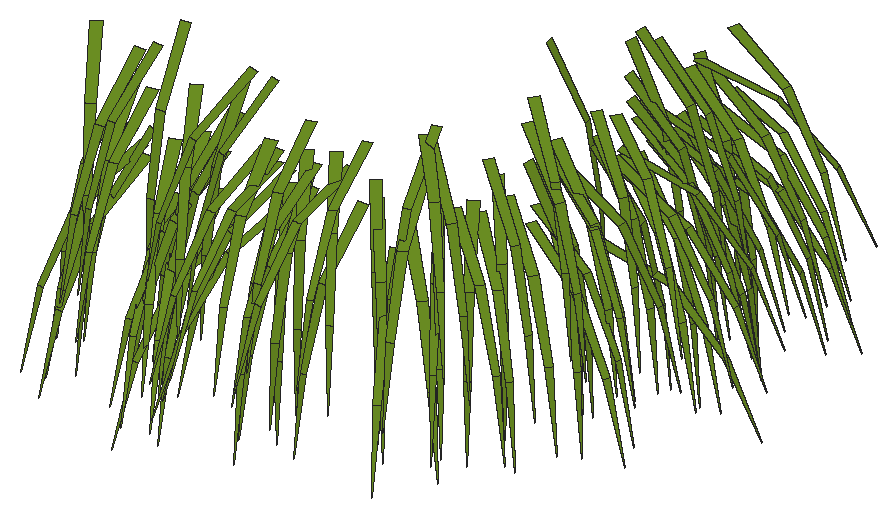
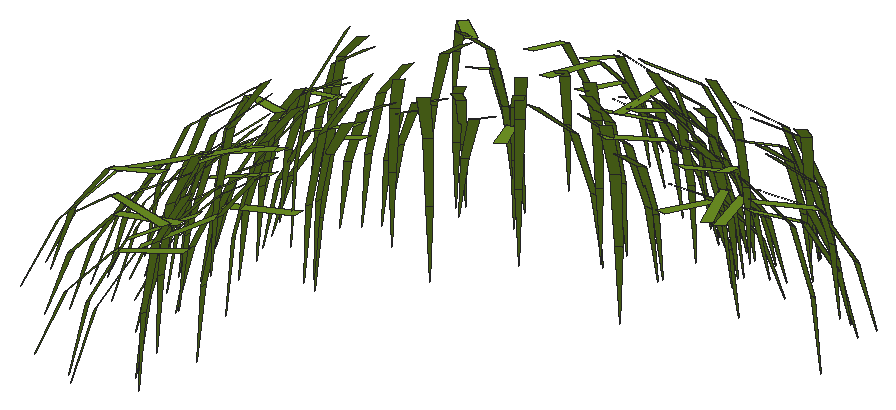
# SketchUp Ruby script. Lengths in inches.
U = 1.inch
M = Sketchup.active_model
def pt(a) = Geom::Point3d.new(a.map { |v| v * U })
def face(e, loops, mat)
  f = e.add_face(loops[0].map { |a| pt(a) })
  loops[1..].each { |l| e.add_face(l.map { |a| pt(a) }).erase! }
  f.material = f.back_material = mat if mat
  f
end
# faces: each face lists its corners as indices into pts; further lists are holes
def faces(e, pts, list, mat = nil) = list.each { |f| face(e, (f[0].is_a?(Array) ? f : [f]).map { |l| l.map { |i| pts[i] } }, mat) }
# xy, xz, yz: faces in a plane at the given z, y or x. An outline is a flat list of corners, or four numbers for a rectangle; further outlines are holes
def ring(l) = l.size == 4 ? [[l[0], l[1]], [l[2], l[1]], [l[2], l[3]], [l[0], l[3]]] : l.each_slice(2).to_a
def flat(e, list, mat, &to3) = list.each { |f| face(e, (f[0].is_a?(Array) ? f : [f]).map { |l| ring(l).map { |u, v| to3.(u, v) } }, mat) }
def xy(e, z, list, mat = nil) = flat(e, list, mat) { |x, y| [x, y, z] }
def xz(e, y, list, mat = nil) = flat(e, list, mat) { |x, z| [x, y, z] }
def yz(e, x, list, mat = nil) = flat(e, list, mat) { |y, z| [x, y, z] }
def lines(e, pts, list) = list.each { |a, b| e.add_line(pt(pts[a]), pt(pts[b])) }
# prism: a flat outline (further loops are holes) pulled along v
def prism(e, loops, v, mat = nil)
  f = face(e, loops, mat); d = Geom::Vector3d.new(v.map { |x| x * U })
  f.pushpull(f.normal.samedirection?(d) ? d.length : -d.length)
end
def box(e, o, s, mat = nil) = prism(e, [[o, [o[0] + s[0], o[1], o[2]], [o[0] + s[0], o[1] + s[1], o[2]], [o[0], o[1] + s[1], o[2]]]], [0, 0, s[2]], mat)
def at(x, y, z, deg = 0) = Geom::Transformation.translation(pt([x, y, z])) * Geom::Transformation.rotation(ORIGIN, Z_AXIS, deg.degrees)
def axes(o, x, y, z) = Geom::Transformation.new([*x, 0, *y, 0, *z, 0, *pt(o).to_a, 1])
def part(name) = M.definitions.add(name)
# library, detail: a bought-in or finely detailed component or shape, given as its bounding box
def library(name, o, s) = part(name).tap { |d| box(d.entities, o, s) }
def detail(e, o, s) = box(e.add_group.entities, o, s)
def put(e, d, t, mat = nil) = e.add_instance(d, t).tap { |i| i.material = mat if mat }
def group(e, t, mat = nil) = e.add_group.tap { |g| g.transformation = t; g.material = mat if mat }.entities
root = M.entities
M.materials.add("[0061_OliveDrab]").color = [107, 142, 35]
p = [[570.33,4.46,549.35],[570.13,4.36,549.35],[570.3,4.27,546.73],[578.04,13.58,549.32],[578.01,13.38,549.32],[578.3,13.43,546.71],
  [567.76,2.63,549.36],[567.58,2.6,549.36],[567.8,2,546.81],[577.62,8.9,549.64],[577.5,8.72,549.64],[577.875,8.6,547.04],
  [578.36,15.74,549.62],[578.36,15.53,549.62],[578.73,15.64,547.02],[567.34,1.68,549.49],[567.14,1.69,549.49],[567.19,0.69,547.06],
  [570.32,2.78,549.65],[570.15,2.71,549.65],[570.51,2.05,547.13],[563.88,3.65,549.66],[563.7,3.71,549.66],[563.71,3.4,547.05],
  [575.6,6.45,549.68],[575.43,6.34,549.68],[575.66,6.18,547.07],[580.17,12.39,549.47],[580.18,12.16,549.47],[581.41,12.33,547.16],
  [578.24,15.81,549.85],[578.24,15.61,549.85],[578.58,15.7,547.25],[579.03,17.18,549.77],[579.1,16.98,549.77],[579.73,17.33,547.24],
  [564.12,2.25,549.77],[563.9,2.27,549.77],[563.95,1.45,547.28],[577.73,16.7,549.91],[577.68,16.5,549.91],[577.91,16.55,547.29],
  [572.05,3.42,550],[571.84,3.41,550],[571.97,2.97,547.42],[579.04,12.85,549.91],[578.99,12.68,549.91],[579.77,12.5625,547.41],
  [570.27,3.16,550.09],[570.04,3.16,550.09],[570.14,2.75,547.49],[579.09,17.45,550.14],[579.13,17.26,550.14],[579.69,17.49,547.59],
  [574.92,3.2,550.09],[574.74,3.09,550.09],[575.37,2.26,547.68],[573.54,4.96,550.3],[573.39,4.83,550.3],[573.6,4.74,547.68],
  [579.03,14.57,550.21],[579.03,14.34,550.21],[579.68,14.45,547.66],[579.96,17.4,550.125],[579.97,17.18,550.125],[581.05,17.32,547.74],
  [563.45,2.23,550.33],[563.23,2.28,550.33],[563.19,1.55,547.81],[564.05,2.47,550.34],[563.83,2.46,550.34],[563.98,1.71,547.82],
  [575.86,4.53,550.27],[575.72,4.36,550.27],[576.51,3.82,547.83],[579.09,8.36,550.21],[579.02,8.16,550.21],[580,7.93,547.79],
  [577.9,12.36,550.37],[577.94,12.15,550.37],[578.17,12.29,547.76],[567.2,1.79,550.24],[567.03,1.72,550.24],[567.6,0.59,547.95],
  [577.34,6.16,550.41],[577.21,5.99,550.41],[577.84,5.64,547.88],[578.93,9.05,550.4375],[578.89,8.87,550.4375],[579.62,8.8,547.92],
  [577.34,9.68,550.47],[577.31,9.46,550.47],[577.53,9.54,547.85],[566.8,2.1,550.51],[566.58,2.11,550.51],[566.67,1.24,548.03],
  [574.41,4.08,550.53],[574.26,3.95,550.53],[574.7,3.59,547.97],[576.52,6.95,550.65],[576.37,6.82,550.65],[576.66,6.65,548.04],
  [577.18,9.46,550.57],[577.16,9.24,550.57],[577.36,9.33,547.96],[579.02,11.88,550.44],[578.93,11.69,550.44],[579.76,11.43,547.96],
  [568.04,1.92,550.33],[567.86,1.82,550.33],[568.57,0.69,548.07],[571.08,3.375,550.67],[570.87,3.3125,550.67],[571.1,2.95,548.08],
  [577.92,7.24,550.63],[577.8,7.05,550.63],[578.45,6.78,548.1],[571.24,4.2,550.8125],[571.05,4.09,550.8125],[571.27,3.94,548.2],
  [567.06,2.41,550.78],[566.84,2.42,550.78],[566.92,1.71,548.25],[567.51,2.95,550.78],[567.3,2.88,550.78],[567.63,2.25,548.25],
  [575.84,4.57,550.78],[575.68,4.46,550.78],[576.23,3.84,548.28],[577.21,5.73,550.75],[577.09,5.55,550.75],[577.85,5.18,548.26],
  [578.26,11.375,550.86],[578.19,11.16,550.86],[578.6,11.15,548.27],[579.89,13.19,550.68],[579.88,12.99,550.68],[581.01,13.0625,548.31],
  [575.91,4.82,550.91],[575.76,4.7,550.91],[576.28,4.23,548.38],[577.45,16.27,551.05],[577.38,16.07,551.05],[577.59,16.12,548.43],
  [568.88,1.85,550.85],[568.68,1.89,550.85],[568.5625,0.79,548.47],[567.23,2.48,550.98],[567.05,2.375,550.98],[567.6,1.55,548.55],
  [578.25,14.02,551.08],[578.25,13.8,551.08],[578.57,13.9,548.48],[563.69,3.07,551.16],[563.5,3.06,551.16],[563.61,2.66,548.5625],
  [567.2,3.62,551.26],[566.99,3.67,551.26],[567.03,3.31,548.66],[577.01,7.42,551.26],[576.92,7.25,551.26],[577.35,7.14,548.67],
  [568.85,2.55,551.31],[568.64,2.57,551.31],[568.68,1.82,548.79],[578.97,10.91,551.37],[578.99,10.6875,551.37],[579.7,10.84,548.84],
  [579.76,12.26,551.29],[579.73,12.05,551.29],[580.64,12.02,548.82],[568.88,2.13,551.35],[568.6875,2.17,551.35],[568.61,1.24,548.89],
  [567.03,3.29,551.45],[566.85,3.32,551.45],[566.89,2.92,548.85],[577.92,11.11,551.53],[577.83,10.93,551.53],[578.16,10.88,548.93],
  [579.27,13.67,551.38],[579.25,13.47,551.38],[580.13,13.52,548.91],[578.53,14,551.52],[578.55,13.8,551.52],[578.97,13.9375,548.9375],
  [579.17,15.17,551.45],[579.22,14.96,551.45],[579.92,15.26,548.9375],[580,17.125,551.27],[579.98,16.91,551.27],[581.02,16.92,548.86],
  [564.84,2.89,551.65],[564.66,2.84,551.65],[564.93,2.27,549.11],[569.875,2.55,551.78],[569.66,2.49,551.78],[569.96,1.86,549.25],
  [574.83,3.89,551.78],[574.62,3.81,551.78],[575,3.21,549.25],[578.37,9.35,551.75],[578.28,9.15,551.75],[578.79,9.04,549.18],
  [579.8125,13.99,551.58],[579.85,13.8,551.58],[580.83,14.1,549.16],[579.35,16.93,551.68],[579.34,16.72,551.68],[580.25,16.76,549.22],
  [570.17,4.88,551.93],[569.89,4.74,551.93],[578.9,9.24,551.86],[578.83,9.05,551.86],[579.56,8.9,549.34],[577.36,13.74,551.85],
  [577.3125,13.47,551.85],[567.56,3.85,551.68],[567.3,3.79,551.68],[573,3.43,551.9],[572.84,3.31,551.9],[573.31,2.83,549.36],
  [567.93,4.15,552.05],[567.72,4.12,552.05],[567.85,3.91,549.43],[579.5625,15.49,551.92],[579.6,15.3,551.92],[580.44,15.57,549.45],
  [565.15,2.36,551.98],[564.95,2.32,551.98],[565.18,1.57,549.47],[567.47,3.41,551.45],[567.19,3.43,551.45],[579.15,8.9,551.9375],
  [579.07,8.72,551.9375],[579.94,8.43,549.48],[578.25,12.35,551.27],[578.27,12.03,551.27],[568.58,1.87,551.98],[568.38,1.87,551.98],
  [568.47,0.83,549.57],[571.04,2.12,552.05],[570.85,2.09,552.05],[571.08,1.27,549.57],[569.88,4.01,551.92],[569.63,3.92,551.92],
  [576.94,9.39,552.125],[576.78,9.13,552.125],[578.24,13.96,552.15],[578.25,13.73,552.15],[578.61,13.86,549.55],[579.3,15.5,552.09],
  [579.25,15.28,552.09],[580.11,15.19,549.61],[577.51,15.78,552.1],[577.51,15.47,552.1],[567.72,3.3,552.25],[567.53,3.1875,552.25],
  [567.92,2.75,549.69],[564.12,4.32,552.1875],[563.87,4.39,552.1875],[575.28,6.99,552.23],[575.04,6.83,552.23],[564.27,3.68,551.97],
  [563.96,3.7,551.97],[576.11,5.64,552.37],[575.99,5.46,552.37],[576.54,5.2,549.8125],[577.76,16.75,552.03],[577.87,16.48,552.03],
  [577.76,13.24,552.18],[577.7,12.99,552.18],[577.3,13.92,552.56],[577.26,13.7,552.56],[577.51,13.77,549.95],[577.45,15.88,552.35],
  [577.44,15.59,552.35],[577.18,16.88,552.47],[577.11,16.61,552.47],[572.03,4.39,552.44],[571.74,4.375,552.44],[574.23,4.7,552.625],
  [574.04,4.65,552.625],[574.25,4.22,550.04],[578.01,8.41,552.54],[577.92,8.22,552.54],[578.48,8.06,549.98],[574.06,4.7,552.0625],
  [573.8,4.55,552.0625],[570.34,4.08,552.54],[570.02,4.09,552.54],[580.23,16.78,552.32],[580.16,16.58,552.32],[581.52,16.26,550.09],
  [577.88,17.22,552.46],[577.94,16.95,552.46],[578.2,17.39,552.07],[578.21,17.09,552.07],[566.47,3.625,551.98],[566.23,3.52,551.98],
  [564.25,2.79,552.69],[564.04,2.77,552.69],[564.21,2.07,550.17],[564.45,3.16,552.78],[564.26,3.17,552.78],[564.35,2.69,550.2],
  [567.99,3.61,552.84],[567.82,3.65,552.84],[567.82,3.25,550.25],[577.5625,8.9375,552.27],[577.47,8.66,552.27],[577.82,14.62,552.53],
  [577.8125,14.3,552.53],[571.61,1.91,552.72],[571.4,1.9,552.72],[571.53,0.78,550.35],[567.13,3.73,552],[566.88,3.6,552],
  [563.79,3.59,552.55],[563.48,3.65,552.55],[564.02,3.81,552.6],[563.71,3.79,552.6],[565.64,4.52,552.95],[565.45,4.47,552.95],
  [565.6,4.25,550.34],[574.73,5.58,552.4],[574.52,5.34,552.4],[573.21,5.41,552.86],[573,5.22,552.86],[577.43,8.59,552.91],
  [577.32,8.42,552.91],[577.77,8.25,550.33],[571.09,2.58,552.96],[570.89,2.52,552.96],[571.1875,1.82,550.45],[564.13,3.57,552.9375],
  [563.95,3.45,552.9375],[564.34,3.07,550.37],[576.31,7.02,552.67],[576.12,6.78,552.67],[577.6,9.39,552.67],[577.54,9.13,552.67],
  [579.36,10.85,552.79],[579.26,10.68,552.79],[580.19,10.24,550.375],[577.74,12.5,552.65],[577.62,12.24,552.65],[577.25,12.31,552.91],
  [577.3,12,552.91],[578.61,14.86,552.96],[578.59,14.67,552.96],[579.18,14.7,550.4],[569.75,1.36,552.77],[569.5625,1.34,552.77],
  [569.84,0,550.53],[572.87,2.68,553.01],[572.6875,2.63,553.01],[572.99,1.8125,550.53],[566.88,3.61,552.66],[566.58,3.61,552.66],
  [573.7,4.96,552.9],[573.49,4.78,552.9],[576.79,9.8125,553.03],[576.74,9.5,553.03],[576.02,7.55,553.16],[575.8125,7.36,553.16],
  [576.83,7.97,552.91],[576.66,7.69,552.91],[576.66,9.55,553.14],[576.63,9.24,553.14],[575.96,11.96,553.17],[576,11.77,553.17],
  [576.13,11.89,550.55],[578.12,14.51,553.21],[578.1,14.29,553.21],[578.58,14.35,550.63],[579.6,17.55,553.04],[579.55,17.33,553.04],
  [580.54,17.22,550.61],[579.57,18.16,552.93],[579.64,17.98,552.93],[580.67,18.46,550.57],[567.04,3.12,553.25],[566.86,3.16,553.25],
  [566.8,2.54,550.7],[566.84,2.64,551.16],[570.84,4.26,553.13],[570.56,4.17,553.13],[576.01,6.57,552.93],[575.85,6.32,552.93],
  [578.14,13.27,552.64],[578.13,12.99,552.64],[567.16,3.73,553.05],[566.85,3.74,553.05],[567.15,4.125,553.11],[566.85,4.02,553.11],
  [570.95,4.75,553.36],[570.6875,4.59,553.36],[575.06,5.74,552.99],[574.84,5.58,552.99],[569.26,3.55,552.82],[568.98,3.61,552.82],
  [575.11,5.83,553.2],[574.9,5.65,553.2],[577.45,11.69,553.34],[577.35,11.38,553.34],[566.52,3.93,553.05],[566.25,3.79,553.05],
  [576.98,16.48,553.625],[576.89,16.2,553.625],[577.47,14.09,553.59],[577.46,13.78,553.59],[563.6875,4,553.61],[563.43,3.99,553.61],
  [576.18,4.51,553.62],[576.02,4.36,553.62],[576.8125,3.71,551.2],[569.21,3.65,553.47],[568.93,3.7,553.47],[569.01,3.85,553.59],
  [568.71,3.88,553.59],[567.41,4.375,553.77],[567.11,4.4375,553.77],[576.21,7.87,553.72],[576.09,7.625,553.72],[575.7,12.27,551.85],
  [575.71,11.88,551.85],[578.18,12.55,553.36],[578.13,12.25,553.36],[578.25,17.33,553.22],[578.22,17.03,553.22],[567.19,4.16,553.92],
  [566.93,4.2,553.92],[577.65,10.875,553.64],[577.67,10.5625,553.64],[577.85,13.79,553.59],[577.84,13.51,553.59],[567.64,5.95,552.1],
  [567.3,5.97,552.1],[577.24,11.48,554.04],[577.12,11.23,554.04],[577.57,13.96,553.97],[577.59,13.67,553.97],[577.84,14.85,553.69],
  [577.91,14.57,553.69],[578.12,13.6875,553.57],[578.18,13.42,553.57],[564.53,4.04,553.99],[564.27,3.97,553.99],[567.16,5.99,553.14],
  [566.84,5.93,553.14],[577.89,17.09,553.86],[577.87,16.79,553.86],[569.55,3.83,554.05],[569.25,3.74,554.05],[574.34,5.15,554.03],
  [574.06,5.02,554.03],[577.39,9.84,554.14],[577.26,9.5625,554.14],[572.3,4.51,554.19],[572.06,4.34,554.19],[569.125,6.02,553.4375],
  [568.82,5.9,553.4375],[569.64,6.04,554.22],[569.3,5.875,554.22],[569.75,5.8125,553.77],[577.72,9.59,554.02],[577.6,9.35,554.02],
  [577.61,9.72,554.1],[577.52,9.45,554.1],[575.74,14.08,553.88],[575.68,13.74,553.88],[578.03,15.22,554.04],[578.09,14.95,554.04],
  [568.64,3.55,554],[568.36,3.55,554],[564.96,3.76,554.19],[564.67,3.71,554.19],[565.49,6.02,552.42],[565.2,5.9,552.42],
  [565.94,6.04,552.37],[565.64,5.88,552.37],[564.47,5.95,553.28],[564.09,5.97,553.28],[567.89,4.74,554.6],[567.59,4.7,554.6],
  [575.64,16,553.38],[575.77,15.66,553.38],[570.84,3.65,554.18],[570.57,3.61,554.18],[572.79,6.85,552.86],[572.47,6.66,552.86],
  [575.49,10.37,554.08],[575.29,10.05,554.08],[577.37,13.97,554.63],[577.38,13.65,554.63],[577.89,15.89,554.27],[577.8125,15.58,554.27],
  [575.7,15.8,554],[575.71,15.43,554],[575.7,17.35,552.87],[575.71,16.98,552.87],[564.61,5.91,554.21],[564.31,6,554.21],
  [574.46,8.25,554.38],[574.17,8.05,554.38],[575.75,13.8125,553.76],[575.66,13.51,553.76],[567.16,4.33,554.6],[566.89,4.17,554.6],
  [575.32,9.75,553.37],[575.2,9.41,553.37],[578.25,17.45,553.91],[578.16,17.17,553.91],[571.96,6.35,554.19],[571.6,6.33,554.19],
  [573.04,7.1,553.71],[572.79,6.8,553.71],[575.16,6.37,554.71],[574.98,6.12,554.71],[575.71,15.97,554.32],[575.7,15.62,554.32],
  [570.43,6.03,554.3],[570.05,6.04,554.3],[576.99,8.95,554.9],[576.86,8.68,554.9],[575.71,14.66,554.1],[575.71,14.27,554.1],
  [575.67,16.75,553.8],[575.74,16.42,553.8],[575.75,17.28,554.63],[575.66,16.94,554.63],[564.33,5.92,553.63],[563.96,6,553.63],
  [563.93,5.97,554.08],[563.5625,5.95,554.08],[574.01,5.71,555.04],[573.75,5.65,555.04],[575.78,13.43,554.13],[575.63,13.1,554.13],
  [575.71,13.36,553.625],[575.7,13.01,553.625],[576.71,14.08,555.11],[576.65,13.76,555.11],[571.61,3.73,554.61],[571.33,3.73,554.61],
  [564.18,4.08,554.98],[563.88,4.05,554.98],[566.97,5.95,553.83],[566.6,5.96,553.83],[574.53,8.45,553.97],[574.3,8.15,553.97],
  [575.34,9.92,553.89],[575.26,9.6,553.89],[569.51,3.4,554.41],[569.25,3.36,554.41],[564.52,4.1875,555.2],[564.24,4.19,555.2],
  [568.24,4.47,555.31],[567.99,4.53,555.31],[569.77,5.92,553.82],[569.43,5.99,553.82],[577.9,11.77,554.77],[577.75,11.52,554.77],
  [563.53,4.53,555.31],[563.28,4.36,555.31],[565.54,5.16,555.49],[565.27,5.1,555.49],[572.33,6.58,554.44],[572.07,6.36,554.44],
  [572.28,6.55,555.03],[572.02,6.33,555.03],[574.11,7.85,554.21],[573.91,7.54,554.21],[574.98,9.15,554.34],[574.77,8.82,554.34],
  [576.63,9.1875,555.34],[576.47,8.95,555.34],[575.68,12.1,555.01],[575.73,11.73,555.01],[577.89,17.57,554.86],[577.98,17.32,554.86],
  [570.77,3.97,555.17],[570.47,3.89,555.17],[572.53,4.2,555.125],[572.27,4.13,555.125],[567.3,5.95,554.44],[566.92,5.97,554.44],
  [565.44,6.04,554.16],[565.12,5.875,554.16],[573.81,7.55,554.42],[573.55,7.37,554.42],[575.35,10.0625,555.22],[575.29,9.68,555.22],
  [577.47,15.03,555.32],[577.44,14.77,555.32],[577.99,17.96,555.07],[577.92,17.65,555.07],[566.52,6.02,554.8],[566.15,5.89,554.8],
  [570.3125,6.07,554.96],[569.96,5.96,554.96],[575.24,9.71,555.35],[575.21,9.33,555.35],[573.73,7.52,554.66],[573.47,7.3,554.66],
  [574.85,8.88,555.09],[574.59,8.64,555.09],[575.53,11.92,555.76],[575.58,11.65,555.76],[577.125,14.66,555.64],[577.09,14.35,555.64],
  [575.72,17.6,553.875],[575.6875,17.23,553.875],[567.38,4.28,555.58],[567.11,4.34,555.58],[575.77,12.27,555.27],[575.65,11.89,555.27],
  [570.16,6.12,555.46],[569.84,5.92,555.46],[575.73,12.96,554.23],[575.68,12.59,554.23],[569.67,5.93,554.68],[569.33,5.99,554.68],
  [569.23,5.94,555.16],[568.86,5.98,555.16],[563.64,5.97,555.34],[563.32,5.96,555.34],[575,5.78,555.6],[574.78,5.56,555.6],
  [575.45,10.78,555.0625],[575.48,10.39,555.0625],[575.67,13.22,554.39],[575.74,12.9,554.39],[575.72,13.9375,555.11],[575.7,13.59,555.11],
  [575.68,14.18,555.5],[575.67,13.79,555.5],[575.66,16.95,555.84],[575.55,16.61,555.84],[574.59,8.73,555.6],[574.43,8.42,555.6],
  [575.66,14.31,555.05],[575.75,13.96,555.05],[567.79,6.01,555.78],[567.43,6.09,555.78],[567.47,6.02,555.75],[567.15,6.06,555.75],
  [575.72,17.28,555.32],[575.69,16.92,555.32],[575.76,18.27,554.11],[575.65,17.92,554.11],[568.7,5.96,555.04],[568.36,5.96,555.04],
  [568.94,6.02,555.36],[568.57,5.91,555.36],[563.94,6.06,555.57],[563.625,5.96,555.57],[573.48,7.28,555.29],[573.12,7.13,555.29],
  [575.51,10.63,555],[575.375,10.33,555],[575.65,12.29,555.97],[575.5,11.98,555.97],[575.61,13.83,555.71],[575.64,13.47,555.71],
  [575.67,14.77,555.08],[575.74,14.43,555.08],[575.46,10.49,555.38],[575.34,10.16,555.38],[575.46,10.75,555.67],[575.3,10.41,555.67],
  [570.5,6.08,555.1],[570.17,6.03,555.1],[564.62,6.02,555.48],[564.26,5.96,555.48],[571.04,6.33,555.6],[570.75,6.125,555.6],
  [575.7,16.45,555.6],[575.61,16.08,555.6],[569.18,5.98,554.75],[568.87,5.9375,554.75],[571.6,6.27,555.26],[571.25,6.27,555.26],
  [566.09,6.21,556.09],[565.75,6.01,556.09],[567.72,6.26,556.73],[567.36,6.21,556.73],[575.48,13.9375,556.44],[575.49,13.54,556.44],
  [573.41,7.65,556.19],[573.2,7.34,556.19],[575.75,13.07,555.54],[575.57,12.77,555.54],[575.09,9.91,556.44],[574.93,9.58,556.44],
  [575.5625,16.74,555.75],[575.68,16.43,555.75],[564.02,6.21,556.5],[563.65,6.18,556.5],[573.52,7.73,556.65],[573.2,7.65,556.65],
  [573.65,7.19,556.22],[571.96,6.57,556.1],[571.64,6.49,556.1],[575.21,14.39,557.25],[575.14,14.01,557.25],[575.61,18.54,556.01],
  [575.53,18.16,556.01],[570.18,6.26,556.29],[569.82,6.17,556.29],[564.6,6.25,556.82],[564.26,6.26,556.82],[562.33,6.35,556.77],
  [562.02,6.14,556.77],[568.72,6.35,557.08],[568.41,6.42,557.08],[575,10.32,557.05],[574.8,10.03,557.05],[575.41,15.3125,556.91],
  [575.37,14.99,556.91],[565.23,6.74,557.57],[564.9,6.67,557.57],[567.9375,6.35,557.09],[567.61,6.43,557.09],[573.28,7.59,556.4],
  [573,7.32,556.4],[575.14,14.91,557.33],[575.1,14.53,557.33],[574.32,11.72,558.08],[574.38,11.4,558.08]]
faces(root,p,[[0,1,2],[3,4,5],[6,7,8],[9,10,11],[12,13,14],[15,16,17],[18,19,20],[21,22,23],
  [24,25,26],[27,28,29],[30,31,32],[33,34,35],[36,37,38],[39,40,41],[42,43,44],[45,46,47],
  [48,49,50],[51,52,53],[54,55,56],[57,58,59],[60,61,62],[63,64,65],[66,67,68],[69,70,71],
  [72,73,74],[75,76,77],[78,79,80],[81,82,83],[84,85,86],[87,88,89],[90,91,92],[93,94,95],
  [96,97,98],[99,100,101],[102,103,104],[105,106,107],[108,109,110],[111,112,113],[114,115,116],[117,118,119],
  [120,121,122],[123,124,125],[126,127,128],[129,130,131],[132,133,134],[135,136,137],[138,139,140],[141,142,143],
  [144,145,146],[147,148,149],[150,151,152],[153,154,155],[156,157,158],[159,160,161],[162,163,164],[165,166,167],
  [168,169,170],[171,172,173],[174,175,176],[177,178,179],[180,181,182],[183,184,185],[186,187,188],[189,190,191],
  [192,193,194],[195,196,197],[198,199,200],[201,202,203],[204,205,206],[207,208,209],[210,211,1,0],[212,213,214],
  [215,216,4,3],[217,218,7,6],[219,220,221],[222,223,224],[225,226,227],[228,229,230],[231,232,16,15],[233,234,235],
  [236,237,28,27],[238,239,240],[241,242,243],[244,245,19,18],[246,247,10,9],[248,249,250],[251,252,253],[254,255,13,12],
  [256,257,258],[259,260,22,21],[261,262,25,24],[263,264,37,36],[265,266,267],[268,269,34,33],[270,271,46,45],[272,273,274],
  [275,276,31,30],[277,278,40,39],[279,280,43,42],[281,282,283],[284,285,286],[287,288,55,54],[289,290,49,48],[291,292,293],
  [294,295,52,51],[296,297,64,63],[298,299,82,81],[300,301,302],[303,304,305],[306,307,308],[309,310,76,75],[311,312,61,60],
  [313,314,315],[316,317,109,108],[318,319,67,66],[320,321,70,69],[322,323,324],[325,326,73,72],[327,328,58,57],[329,330,331],
  [332,333,334],[335,336,337],[338,339,85,84],[340,341,88,87],[342,343,344],[345,346,106,105],[347,348,79,78],[349,350,351],
  [352,353,354],[355,356,357],[358,359,94,93],[360,361,97,96],[362,363,91,90],[364,365,100,99],[366,367,115,114],[368,369,103,102],
  [370,371,372],[373,374,375],[376,377,378],[379,380,381],[382,383,384,385],[386,387,112,111],[388,389,130,129],[390,391,136,135],
  [392,393,385,121,120],[394,395,124,123],[396,397,118,117],[398,399,127,126],[400,401,145,144],[402,403,139,138],[404,405,133,132],[406,407,148,147],
  [408,409,142,141],[410,411,151,150],[412,413,154,153],[414,415,416],[417,418,172,171],[419,420,163,162],[421,422,157,156],[423,424,160,159],
  [425,426,237,236],[427,428,169,168],[429,430,190,189],[431,432,175,174],[433,434,166,165],[435,436,181,180],[437,438,232,231],[439,440,178,177],
  [441,442,184,183],[443,444,187,186],[445,446,205,204],[447,448,193,192],[449,450,218,217],[451,452,208,207],[453,454,196,195],[455,456,199,198],
  [457,458,202,201],[459,460,220,219],[461,462,245,244],[463,464,211,210,465],[466,467,234,233],[468,469,213,212],[470,471,216,215],[472,473,226,225],
  [474,475,239,238],[476,477,229,228],[478,479,299,298],[480,481,317,316],[482,483,264,263],[484,485,223,222],[486,487,269,268],[488,489,242,241],
  [490,491,288,287],[492,493,247,246],[494,495,249,248],[496,497,252,251],[498,499,255,254],[500,501,297,296],[502,503,260,259],[504,505,262,261],
  [506,507,271,270],[508,509,257,256],[510,511,310,309],[512,513,292,291],[514,515,280,279],[516,517,326,325],[518,519,266,265],[520,521,276,275],
  [522,523,290,289],[524,525,285,284],[526,527,312,311],[528,529,295,294],[530,531,278,277],[532,533,319,318],[534,535,321,320],[536,537,282,281],
  [538,539,346,345],[540,541,391,390],[542,543,273,272],[544,545,314,313],[546,547,301,300],[548,549,359,358],[550,551,339,338],[552,553,341,340],
  [554,555,353,352],[556,557,304,303],[558,559,307,306],[560,561,401,400,465],[562,563,343,342],[564,565,336,335],[566,567,323,322],[568,569,361,360],
  [570,571,328,327],[572,573,389,388],[574,575,367,366],[576,577,330,329],[578,579,348,347],[580,581,380,379],[582,583,333,332],[584,585,356,355],
  [586,587,393,392],[588,589,407,406],[590,591,399,398],[592,593,363,362],[594,595,350,349],[596,597,377,376],[598,599,395,394],[600,601,387,386],
  [602,603,369,368],[604,605,403,402],[606,607,365,364],[608,609,371,370],[610,611,374,373],[612,613,430,429],[614,615,383,382],[616,617,405,404],
  [618,619,397,396],[620,621,428,427],[622,623,418,417],[624,625,420,419],[626,627,413,412],[628,629,415,414],[630,631,434,433],[632,633,446,445],
  [634,635,436,435],[636,637,411,410],[638,639,409,408],[640,641,424,423],[642,643,444,443],[644,645,422,421],[646,647,432,431],[648,649,452,451],
  [650,651,513,512],[652,653,475,474],[654,655,454,453],[656,657,448,447],[658,659,456,455],[660,661,467,466],[662,663,440,439],[664,665,442,441],
  [666,667,473,472],[668,669,469,468],[670,671,458,457],[672,673,489,488],[674,675,477,476],[676,677,460,459],[678,679,497,496],[680,681,555,554],
  [682,683,545,544],[684,685,509,508],[686,687,485,484],[688,689,495,494],[690,691,519,518],[692,693,563,562],[694,695,525,524],[696,697,581,580],
  [698,699,547,546],[700,701,537,536,702],[703,704,585,584],[705,706,543,542],[707,708,597,596],[709,710,583,582],[711,712,557,556],[713,714,565,564],
  [715,716,559,558],[717,718,577,576],[719,720,595,594],[721,722,567,566],[723,724,615,614],[725,726,629,628,702],[727,728,611,610],[729,730,609,608]],"[0061_OliveDrab]")
